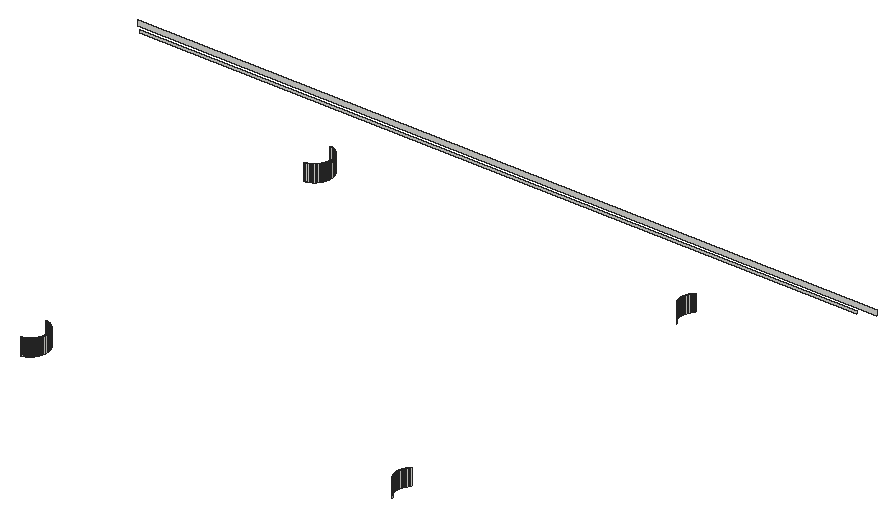
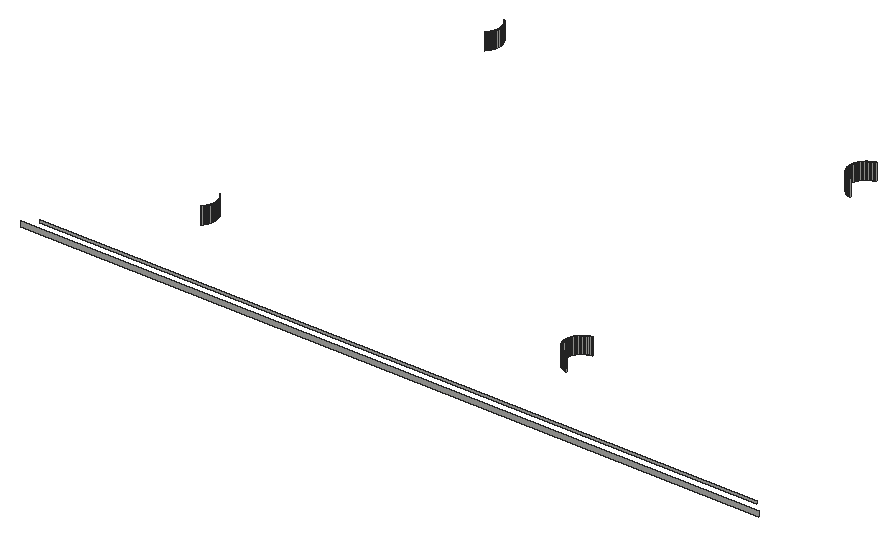
# SketchUp Ruby script. Lengths in inches.
U = 1.inch
M = Sketchup.active_model
def pt(a) = Geom::Point3d.new(a.map { |v| v * U })
def face(e, loops, mat)
  f = e.add_face(loops[0].map { |a| pt(a) })
  loops[1..].each { |l| e.add_face(l.map { |a| pt(a) }).erase! }
  f.material = f.back_material = mat if mat
  f
end
# faces: each face lists its corners as indices into pts; further lists are holes
def faces(e, pts, list, mat = nil) = list.each { |f| face(e, (f[0].is_a?(Array) ? f : [f]).map { |l| l.map { |i| pts[i] } }, mat) }
# xy, xz, yz: faces in a plane at the given z, y or x. An outline is a flat list of corners, or four numbers for a rectangle; further outlines are holes
def ring(l) = l.size == 4 ? [[l[0], l[1]], [l[2], l[1]], [l[2], l[3]], [l[0], l[3]]] : l.each_slice(2).to_a
def flat(e, list, mat, &to3) = list.each { |f| face(e, (f[0].is_a?(Array) ? f : [f]).map { |l| ring(l).map { |u, v| to3.(u, v) } }, mat) }
def xy(e, z, list, mat = nil) = flat(e, list, mat) { |x, y| [x, y, z] }
def xz(e, y, list, mat = nil) = flat(e, list, mat) { |x, z| [x, y, z] }
def yz(e, x, list, mat = nil) = flat(e, list, mat) { |y, z| [x, y, z] }
def lines(e, pts, list) = list.each { |a, b| e.add_line(pt(pts[a]), pt(pts[b])) }
# prism: a flat outline (further loops are holes) pulled along v
def prism(e, loops, v, mat = nil)
  f = face(e, loops, mat); d = Geom::Vector3d.new(v.map { |x| x * U })
  f.pushpull(f.normal.samedirection?(d) ? d.length : -d.length)
end
def box(e, o, s, mat = nil) = prism(e, [[o, [o[0] + s[0], o[1], o[2]], [o[0] + s[0], o[1] + s[1], o[2]], [o[0], o[1] + s[1], o[2]]]], [0, 0, s[2]], mat)
def at(x, y, z, deg = 0) = Geom::Transformation.translation(pt([x, y, z])) * Geom::Transformation.rotation(ORIGIN, Z_AXIS, deg.degrees)
def axes(o, x, y, z) = Geom::Transformation.new([*x, 0, *y, 0, *z, 0, *pt(o).to_a, 1])
def part(name) = M.definitions.add(name)
# library, detail: a bought-in or finely detailed component or shape, given as its bounding box
def library(name, o, s) = part(name).tap { |d| box(d.entities, o, s) }
def detail(e, o, s) = box(e.add_group.entities, o, s)
def put(e, d, t, mat = nil) = e.add_instance(d, t).tap { |i| i.material = mat if mat }
def group(e, t, mat = nil) = e.add_group.tap { |g| g.transformation = t; g.material = mat if mat }.entities
root = M.entities
xz(root,333,[[215,108,345,108.5]])
xz(root,335,[[213,107.5,347,108.5]])
yz(root,262.5,[[252.34,108,252.42,111],[252.42,108,252.5,111],[252.5,108,252.58,111],[252.58,108,252.66,111],[316.84,108,316.92,111],
  [316.92,108,317,111],[317,108,317.08,111],[317.08,108,317.16,111]])
yz(root,326,[[252.34,108,252.42,111],[252.42,108,252.5,111],[252.5,108,252.58,111],[252.58,108,252.66,111],[316.84,108,316.92,111],
  [316.92,108,317,111],[317,108,317.08,111],[317.08,108,317.16,111]])
p = [[260.125,249.57,108],[260.05,249.55,108],[260.05,249.55,111],[260.125,249.57,111],[260.2,249.58,108],[260.2,249.58,111],
  [260.28,249.6,108],[260.28,249.6,111],[260.35,249.625,108],[260.35,249.625,111],[260.43,249.65,108],[260.43,249.65,111],
  [260.5,249.67,108],[260.5,249.67,111],[260.58,249.7,108],[260.58,249.7,111],[260.65,249.73,108],[260.65,249.73,111],
  [260.72,249.76,108],[260.72,249.76,111],[260.79,249.79,108],[260.79,249.79,111],[260.86,249.83,108],[260.86,249.83,111],
  [260.93,249.86,108],[260.93,249.86,111],[261,249.9,108],[261,249.9,111],[261.07,249.94,108],[261.07,249.94,111],
  [261.13,249.98,108],[261.13,249.98,111],[261.2,250.03,108],[261.2,250.03,111],[261.26,250.07,108],[261.26,250.07,111],
  [261.33,250.12,108],[261.33,250.12,111],[261.39,250.17,108],[261.39,250.17,111],[261.45,250.22,108],[261.45,250.22,111],
  [261.51,250.27,108],[261.51,250.27,111],[261.57,250.32,108],[261.57,250.32,111],[261.62,250.38,108],[261.62,250.38,111],
  [326.93,250.32,108],[326.88,250.38,108],[326.88,250.38,111],[326.93,250.32,111],[261.68,250.43,108],[261.68,250.43,111],
  [261.73,250.49,108],[261.73,250.49,111],[326.82,250.43,108],[326.77,250.49,108],[326.77,250.49,111],[326.82,250.43,111],
  [261.78,250.55,108],[261.78,250.55,111],[326.72,250.55,108],[326.72,250.55,111],[261.83,250.61,108],[261.83,250.61,111],
  [261.88,250.67,108],[261.88,250.67,111],[326.67,250.61,108],[326.62,250.67,108],[326.62,250.67,111],[326.67,250.61,111],
  [261.93,250.74,108],[261.93,250.74,111],[261.97,250.8,108],[261.97,250.8,111],[326.57,250.74,108],[326.53,250.8,108],
  [326.53,250.8,111],[326.57,250.74,111],[262.02,250.87,108],[262.02,250.87,111],[326.48,250.87,108],[326.48,250.87,111],
  [262.06,250.93,108],[262.06,250.93,111],[262.1,251,108],[262.1,251,111],[326.44,250.93,108],[326.4,251,108],
  [326.4,251,111],[326.44,250.93,111],[262.14,251.07,108],[262.14,251.07,111],[326.36,251.07,108],[326.36,251.07,111],
  [262.17,251.14,108],[262.17,251.14,111],[262.21,251.21,108],[262.21,251.21,111],[326.33,251.14,108],[326.29,251.21,108],
  [326.29,251.21,111],[326.33,251.14,111],[262.24,251.28,108],[262.24,251.28,111],[326.26,251.28,108],[326.26,251.28,111],
  [262.27,251.35,108],[262.27,251.35,111],[326.23,251.35,108],[326.23,251.35,111],[262.3,251.42,108],[262.3,251.42,111],
  [262.33,251.5,108],[262.33,251.5,111],[326.2,251.42,108],[326.17,251.5,108],[326.17,251.5,111],[326.2,251.42,111],
  [262.35,251.57,108],[262.35,251.57,111],[326.15,251.57,108],[326.15,251.57,111],[262.375,251.65,108],[262.375,251.65,111],
  [262.4,251.72,108],[262.4,251.72,111],[326.125,251.65,108],[326.1,251.72,108],[326.1,251.72,111],[326.125,251.65,111],
  [262.42,251.8,108],[262.42,251.8,111],[326.08,251.8,108],[326.08,251.8,111],[262.43,251.875,108],[262.43,251.875,111],
  [326.07,251.875,108],[326.07,251.875,111],[262.45,251.95,108],[262.45,251.95,111],[326.05,251.95,108],[326.05,251.95,111],
  [262.46,252.03,108],[262.46,252.03,111],[262.47,252.11,108],[262.47,252.11,111],[326.04,252.03,108],[326.03,252.11,108],
  [326.03,252.11,111],[326.04,252.03,111],[262.48,252.1875,108],[262.48,252.1875,111],[326.02,252.1875,108],[326.02,252.1875,111],
  [262.49,252.26,108],[262.49,252.26,111],[326.01,252.26,108],[326.01,252.26,111],[262.5,252.34,108],[262.5,252.34,111],
  [326,252.34,108],[326,252.34,111],[262.48,252.8125,108],[262.49,252.74,108],[262.49,252.74,111],[262.48,252.8125,111],
  [262.5,252.66,108],[262.5,252.66,111],[326,252.66,108],[326.01,252.74,108],[326.01,252.74,111],[326,252.66,111],
  [326.02,252.8125,108],[326.02,252.8125,111],[262.47,252.89,108],[262.47,252.89,111],[326.03,252.89,108],[326.03,252.89,111],
  [262.46,252.97,108],[262.46,252.97,111],[326.04,252.97,108],[326.04,252.97,111],[262.43,253.125,108],[262.45,253.05,108],
  [262.45,253.05,111],[262.43,253.125,111],[326.05,253.05,108],[326.05,253.05,111],[326.07,253.125,108],[326.07,253.125,111],
  [262.42,253.2,108],[262.42,253.2,111],[326.08,253.2,108],[326.08,253.2,111],[262.4,253.28,108],[262.4,253.28,111],
  [326.1,253.28,108],[326.1,253.28,111],[262.375,253.35,108],[262.375,253.35,111],[326.125,253.35,108],[326.125,253.35,111],
  [262.33,253.5,108],[262.35,253.43,108],[262.35,253.43,111],[262.33,253.5,111],[326.15,253.43,108],[326.15,253.43,111],
  [326.17,253.5,108],[326.17,253.5,111],[262.3,253.58,108],[262.3,253.58,111],[326.2,253.58,108],[326.2,253.58,111],
  [262.24,253.72,108],[262.27,253.65,108],[262.27,253.65,111],[262.24,253.72,111],[326.23,253.65,108],[326.23,253.65,111],
  [326.26,253.72,108],[326.26,253.72,111],[262.21,253.79,108],[262.21,253.79,111],[326.29,253.79,108],[326.29,253.79,111],
  [262.17,253.86,108],[262.17,253.86,111],[326.33,253.86,108],[326.33,253.86,111],[262.1,254,108],[262.14,253.93,108],
  [262.14,253.93,111],[262.1,254,111],[326.36,253.93,108],[326.36,253.93,111],[326.4,254,108],[326.4,254,111],
  [262.06,254.07,108],[262.06,254.07,111],[326.44,254.07,108],[326.44,254.07,111],[261.97,254.2,108],[262.02,254.13,108],
  [262.02,254.13,111],[261.97,254.2,111],[326.48,254.13,108],[326.48,254.13,111],[326.53,254.2,108],[326.53,254.2,111],
  [261.93,254.26,108],[261.93,254.26,111],[326.57,254.26,108],[326.57,254.26,111],[261.83,254.39,108],[261.88,254.33,108],
  [261.88,254.33,111],[261.83,254.39,111],[326.62,254.33,108],[326.62,254.33,111],[326.67,254.39,108],[326.67,254.39,111],
  [261.73,254.51,108],[261.78,254.45,108],[261.78,254.45,111],[261.73,254.51,111],[326.72,254.45,108],[326.72,254.45,111],
  [326.77,254.51,108],[326.77,254.51,111],[261.68,254.57,108],[261.68,254.57,111],[326.82,254.57,108],[326.82,254.57,111],
  [261.57,254.68,108],[261.62,254.62,108],[261.62,254.62,111],[261.57,254.68,111],[326.88,254.62,108],[326.88,254.62,111],
  [326.93,254.68,108],[326.93,254.68,111],[261.45,254.78,108],[261.51,254.73,108],[261.51,254.73,111],[261.45,254.78,111],
  [261.33,254.88,108],[261.39,254.83,108],[261.39,254.83,111],[261.33,254.88,111],[261.2,254.97,108],[261.26,254.93,108],
  [261.26,254.93,111],[261.2,254.97,111],[261.07,255.06,108],[261.13,255.02,108],[261.13,255.02,111],[261.07,255.06,111],
  [260.86,255.17,108],[260.93,255.14,108],[260.93,255.14,111],[260.86,255.17,111],[261,255.1,108],[261,255.1,111],
  [260.65,255.27,108],[260.72,255.24,108],[260.72,255.24,111],[260.65,255.27,111],[260.79,255.21,108],[260.79,255.21,111],
  [260.43,255.35,108],[260.5,255.33,108],[260.5,255.33,111],[260.43,255.35,111],[260.58,255.3,108],[260.58,255.3,111],
  [259.97,255.46,108],[260.05,255.45,108],[260.05,255.45,111],[259.97,255.46,111],[260.125,255.43,108],[260.125,255.43,111],
  [260.2,255.42,108],[260.2,255.42,111],[260.28,255.4,108],[260.28,255.4,111],[260.35,255.375,108],[260.35,255.375,111],
  [259.97,314.04,108],[259.89,314.03,108],[259.89,314.03,111],[259.97,314.04,111],[260.05,314.05,108],[260.05,314.05,111],
  [260.125,314.07,108],[260.125,314.07,111],[260.2,314.08,108],[260.2,314.08,111],[260.28,314.1,108],[260.28,314.1,111],
  [260.35,314.125,108],[260.35,314.125,111],[260.43,314.15,108],[260.43,314.15,111],[260.5,314.17,108],[260.5,314.17,111],
  [260.58,314.2,108],[260.58,314.2,111],[260.65,314.23,108],[260.65,314.23,111],[260.72,314.26,108],[260.72,314.26,111],
  [260.79,314.29,108],[260.79,314.29,111],[260.86,314.33,108],[260.86,314.33,111],[260.93,314.36,108],[260.93,314.36,111],
  [261,314.4,108],[261,314.4,111],[261.07,314.44,108],[261.07,314.44,111],[261.13,314.48,108],[261.13,314.48,111],
  [261.2,314.53,108],[261.2,314.53,111],[261.26,314.57,108],[261.26,314.57,111],[261.33,314.62,108],[261.33,314.62,111],
  [261.39,314.67,108],[261.39,314.67,111],[261.45,314.72,108],[261.45,314.72,111],[261.51,314.77,108],[261.51,314.77,111],
  [261.57,314.82,108],[261.57,314.82,111],[261.62,314.88,108],[261.62,314.88,111],[326.93,314.82,108],[326.88,314.88,108],
  [326.88,314.88,111],[326.93,314.82,111],[261.68,314.93,108],[261.68,314.93,111],[261.73,314.99,108],[261.73,314.99,111],
  [326.82,314.93,108],[326.77,314.99,108],[326.77,314.99,111],[326.82,314.93,111],[261.78,315.05,108],[261.78,315.05,111],
  [326.72,315.05,108],[326.72,315.05,111],[261.83,315.11,108],[261.83,315.11,111],[261.88,315.17,108],[261.88,315.17,111],
  [326.67,315.11,108],[326.62,315.17,108],[326.62,315.17,111],[326.67,315.11,111],[261.93,315.24,108],[261.93,315.24,111],
  [261.97,315.3,108],[261.97,315.3,111],[326.57,315.24,108],[326.53,315.3,108],[326.53,315.3,111],[326.57,315.24,111],
  [262.02,315.37,108],[262.02,315.37,111],[326.48,315.37,108],[326.48,315.37,111],[262.06,315.43,108],[262.06,315.43,111],
  [262.1,315.5,108],[262.1,315.5,111],[326.44,315.43,108],[326.4,315.5,108],[326.4,315.5,111],[326.44,315.43,111],
  [262.14,315.57,108],[262.14,315.57,111],[326.36,315.57,108],[326.36,315.57,111],[262.17,315.64,108],[262.17,315.64,111],
  [262.21,315.71,108],[262.21,315.71,111],[326.33,315.64,108],[326.29,315.71,108],[326.29,315.71,111],[326.33,315.64,111],
  [262.24,315.78,108],[262.24,315.78,111],[326.26,315.78,108],[326.26,315.78,111],[262.27,315.85,108],[262.27,315.85,111],
  [326.23,315.85,108],[326.23,315.85,111],[262.3,315.92,108],[262.3,315.92,111],[262.33,316,108],[262.33,316,111],
  [326.2,315.92,108],[326.17,316,108],[326.17,316,111],[326.2,315.92,111],[262.35,316.07,108],[262.35,316.07,111],
  [326.15,316.07,108],[326.15,316.07,111],[262.375,316.15,108],[262.375,316.15,111],[262.4,316.22,108],[262.4,316.22,111],
  [326.125,316.15,108],[326.1,316.22,108],[326.1,316.22,111],[326.125,316.15,111],[262.42,316.3,108],[262.42,316.3,111],
  [326.08,316.3,108],[326.08,316.3,111],[262.43,316.375,108],[262.43,316.375,111],[326.07,316.375,108],[326.07,316.375,111],
  [262.45,316.45,108],[262.45,316.45,111],[326.05,316.45,108],[326.05,316.45,111],[262.46,316.53,108],[262.46,316.53,111],
  [262.47,316.61,108],[262.47,316.61,111],[326.04,316.53,108],[326.03,316.61,108],[326.03,316.61,111],[326.04,316.53,111],
  [262.48,316.6875,108],[262.48,316.6875,111],[326.02,316.6875,108],[326.02,316.6875,111],[262.49,316.76,108],[262.49,316.76,111],
  [326.01,316.76,108],[326.01,316.76,111],[262.5,316.84,108],[262.5,316.84,111],[326,316.84,108],[326,316.84,111],
  [262.48,317.3125,108],[262.49,317.24,108],[262.49,317.24,111],[262.48,317.3125,111],[262.5,317.16,108],[262.5,317.16,111],
  [326,317.16,108],[326.01,317.24,108],[326.01,317.24,111],[326,317.16,111],[326.02,317.3125,108],[326.02,317.3125,111],
  [262.47,317.39,108],[262.47,317.39,111],[326.03,317.39,108],[326.03,317.39,111],[262.46,317.47,108],[262.46,317.47,111],
  [326.04,317.47,108],[326.04,317.47,111],[262.43,317.625,108],[262.45,317.55,108],[262.45,317.55,111],[262.43,317.625,111],
  [326.05,317.55,108],[326.05,317.55,111],[326.07,317.625,108],[326.07,317.625,111],[262.42,317.7,108],[262.42,317.7,111],
  [326.08,317.7,108],[326.08,317.7,111],[262.4,317.78,108],[262.4,317.78,111],[326.1,317.78,108],[326.1,317.78,111],
  [262.375,317.85,108],[262.375,317.85,111],[326.125,317.85,108],[326.125,317.85,111],[262.33,318,108],[262.35,317.93,108],
  [262.35,317.93,111],[262.33,318,111],[326.15,317.93,108],[326.15,317.93,111],[326.17,318,108],[326.17,318,111],
  [262.3,318.08,108],[262.3,318.08,111],[326.2,318.08,108],[326.2,318.08,111],[262.24,318.22,108],[262.27,318.15,108],
  [262.27,318.15,111],[262.24,318.22,111],[326.23,318.15,108],[326.23,318.15,111],[326.26,318.22,108],[326.26,318.22,111],
  [262.21,318.29,108],[262.21,318.29,111],[326.29,318.29,108],[326.29,318.29,111],[262.17,318.36,108],[262.17,318.36,111],
  [326.33,318.36,108],[326.33,318.36,111],[262.1,318.5,108],[262.14,318.43,108],[262.14,318.43,111],[262.1,318.5,111],
  [326.36,318.43,108],[326.36,318.43,111],[326.4,318.5,108],[326.4,318.5,111],[262.06,318.57,108],[262.06,318.57,111],
  [326.44,318.57,108],[326.44,318.57,111],[261.97,318.7,108],[262.02,318.63,108],[262.02,318.63,111],[261.97,318.7,111],
  [326.48,318.63,108],[326.48,318.63,111],[326.53,318.7,108],[326.53,318.7,111],[261.93,318.76,108],[261.93,318.76,111],
  [326.57,318.76,108],[326.57,318.76,111],[261.83,318.89,108],[261.88,318.83,108],[261.88,318.83,111],[261.83,318.89,111],
  [326.62,318.83,108],[326.62,318.83,111],[326.67,318.89,108],[326.67,318.89,111],[261.73,319.01,108],[261.78,318.95,108],
  [261.78,318.95,111],[261.73,319.01,111],[326.72,318.95,108],[326.72,318.95,111],[326.77,319.01,108],[326.77,319.01,111],
  [261.68,319.07,108],[261.68,319.07,111],[326.82,319.07,108],[326.82,319.07,111],[261.57,319.18,108],[261.62,319.12,108],
  [261.62,319.12,111],[261.57,319.18,111],[326.88,319.12,108],[326.88,319.12,111],[326.93,319.18,108],[326.93,319.18,111],
  [261.45,319.28,108],[261.51,319.23,108],[261.51,319.23,111],[261.45,319.28,111],[261.33,319.38,108],[261.39,319.33,108],
  [261.39,319.33,111],[261.33,319.38,111],[261.2,319.47,108],[261.26,319.43,108],[261.26,319.43,111],[261.2,319.47,111],
  [261.07,319.56,108],[261.13,319.52,108],[261.13,319.52,111],[261.07,319.56,111],[260.86,319.67,108],[260.93,319.64,108],
  [260.93,319.64,111],[260.86,319.67,111],[261,319.6,108],[261,319.6,111],[260.65,319.77,108],[260.72,319.74,108],
  [260.72,319.74,111],[260.65,319.77,111],[260.79,319.71,108],[260.79,319.71,111],[260.43,319.85,108],[260.5,319.83,108],
  [260.5,319.83,111],[260.43,319.85,111],[260.58,319.8,108],[260.58,319.8,111],[259.97,319.96,108],[260.05,319.95,108],
  [260.05,319.95,111],[259.97,319.96,111],[260.125,319.93,108],[260.125,319.93,111],[260.2,319.92,108],[260.2,319.92,111],
  [260.28,319.9,108],[260.28,319.9,111],[260.35,319.875,108],[260.35,319.875,111],[259.89,319.97,108],[259.89,319.97,111]]
faces(root,p,[[0,1,2,3],[4,0,3,5],[6,4,5,7],[8,6,7,9],[10,8,9,11],[12,10,11,13],[14,12,13,15],[16,14,15,17],
  [18,16,17,19],[20,18,19,21],[22,20,21,23],[24,22,23,25],[26,24,25,27],[28,26,27,29],[30,28,29,31],[32,30,31,33],
  [34,32,33,35],[36,34,35,37],[38,36,37,39],[40,38,39,41],[42,40,41,43],[44,42,43,45],[46,44,45,47],[48,49,50,51],
  [52,46,47,53],[54,52,53,55],[56,57,58,59],[49,56,59,50],[60,54,55,61],[57,62,63,58],[64,60,61,65],[66,64,65,67],
  [68,69,70,71],[62,68,71,63],[72,66,67,73],[74,72,73,75],[76,77,78,79],[69,76,79,70],[80,74,75,81],[77,82,83,78],
  [84,80,81,85],[86,84,85,87],[88,89,90,91],[82,88,91,83],[92,86,87,93],[89,94,95,90],[96,92,93,97],[98,96,97,99],
  [100,101,102,103],[94,100,103,95],[104,98,99,105],[101,106,107,102],[108,104,105,109],[106,110,111,107],[112,108,109,113],[114,112,113,115],
  [116,117,118,119],[110,116,119,111],[120,114,115,121],[117,122,123,118],[124,120,121,125],[126,124,125,127],[128,129,130,131],[122,128,131,123],
  [132,126,127,133],[129,134,135,130],[136,132,133,137],[134,138,139,135],[140,136,137,141],[138,142,143,139],[144,140,141,145],[146,144,145,147],
  [148,149,150,151],[142,148,151,143],[152,146,147,153],[149,154,155,150],[156,152,153,157],[154,158,159,155],[160,156,157,161],[158,162,163,159],
  [164,165,166,167],[165,168,169,166],[170,171,172,173],[171,174,175,172],[176,164,167,177],[174,178,179,175],[180,176,177,181],[178,182,183,179],
  [184,185,186,187],[185,180,181,186],[182,188,189,183],[188,190,191,189],[192,184,187,193],[190,194,195,191],[196,192,193,197],[194,198,199,195],
  [200,196,197,201],[198,202,203,199],[204,205,206,207],[205,200,201,206],[202,208,209,203],[208,210,211,209],[212,204,207,213],[210,214,215,211],
  [216,217,218,219],[217,212,213,218],[214,220,221,215],[220,222,223,221],[224,216,219,225],[222,226,227,223],[228,224,225,229],[226,230,231,227],
  [232,233,234,235],[233,228,229,234],[230,236,237,231],[236,238,239,237],[240,232,235,241],[238,242,243,239],[244,245,246,247],[245,240,241,246],
  [242,248,249,243],[248,250,251,249],[252,244,247,253],[250,254,255,251],[256,257,258,259],[257,252,253,258],[254,260,261,255],[260,262,263,261],
  [264,265,266,267],[265,256,259,266],[262,268,269,263],[268,270,271,269],[272,264,267,273],[270,274,275,271],[276,277,278,279],[277,272,273,278],
  [274,280,281,275],[280,282,283,281],[284,285,286,287],[285,276,279,286],[288,289,290,291],[289,284,287,290],[292,293,294,295],[293,288,291,294],
  [296,297,298,299],[297,292,295,298],[300,301,302,303],[301,304,305,302],[304,296,299,305],[306,307,308,309],[307,310,311,308],[310,300,303,311],
  [312,313,314,315],[313,316,317,314],[316,306,309,317],[318,319,320,321],[319,322,323,320],[322,324,325,323],[324,326,327,325],[326,328,329,327],
  [328,312,315,329],[330,331,332,333],[334,330,333,335],[336,334,335,337],[338,336,337,339],[340,338,339,341],[342,340,341,343],[344,342,343,345],
  [346,344,345,347],[348,346,347,349],[350,348,349,351],[352,350,351,353],[354,352,353,355],[356,354,355,357],[358,356,357,359],[360,358,359,361],
  [362,360,361,363],[364,362,363,365],[366,364,365,367],[368,366,367,369],[370,368,369,371],[372,370,371,373],[374,372,373,375],[376,374,375,377],
  [378,376,377,379],[380,378,379,381],[382,383,384,385],[386,380,381,387],[388,386,387,389],[390,391,392,393],[383,390,393,384],[394,388,389,395],
  [391,396,397,392],[398,394,395,399],[400,398,399,401],[402,403,404,405],[396,402,405,397],[406,400,401,407],[408,406,407,409],[410,411,412,413],
  [403,410,413,404],[414,408,409,415],[411,416,417,412],[418,414,415,419],[420,418,419,421],[422,423,424,425],[416,422,425,417],[426,420,421,427],
  [423,428,429,424],[430,426,427,431],[432,430,431,433],[434,435,436,437],[428,434,437,429],[438,432,433,439],[435,440,441,436],[442,438,439,443],
  [440,444,445,441],[446,442,443,447],[448,446,447,449],[450,451,452,453],[444,450,453,445],[454,448,449,455],[451,456,457,452],[458,454,455,459],
  [460,458,459,461],[462,463,464,465],[456,462,465,457],[466,460,461,467],[463,468,469,464],[470,466,467,471],[468,472,473,469],[474,470,471,475],
  [472,476,477,473],[478,474,475,479],[480,478,479,481],[482,483,484,485],[476,482,485,477],[486,480,481,487],[483,488,489,484],[490,486,487,491],
  [488,492,493,489],[494,490,491,495],[492,496,497,493],[498,499,500,501],[499,502,503,500],[504,505,506,507],[505,508,509,506],[510,498,501,511],
  [508,512,513,509],[514,510,511,515],[512,516,517,513],[518,519,520,521],[519,514,515,520],[516,522,523,517],[522,524,525,523],[526,518,521,527],
  [524,528,529,525],[530,526,527,531],[528,532,533,529],[534,530,531,535],[532,536,537,533],[538,539,540,541],[539,534,535,540],[536,542,543,537],
  [542,544,545,543],[546,538,541,547],[544,548,549,545],[550,551,552,553],[551,546,547,552],[548,554,555,549],[554,556,557,555],[558,550,553,559],
  [556,560,561,557],[562,558,559,563],[560,564,565,561],[566,567,568,569],[567,562,563,568],[564,570,571,565],[570,572,573,571],[574,566,569,575],
  [572,576,577,573],[578,579,580,581],[579,574,575,580],[576,582,583,577],[582,584,585,583],[586,578,581,587],[584,588,589,585],[590,591,592,593],
  [591,586,587,592],[588,594,595,589],[594,596,597,595],[598,599,600,601],[599,590,593,600],[596,602,603,597],[602,604,605,603],[606,598,601,607],
  [604,608,609,605],[610,611,612,613],[611,606,607,612],[608,614,615,609],[614,616,617,615],[618,619,620,621],[619,610,613,620],[622,623,624,625],
  [623,618,621,624],[626,627,628,629],[627,622,625,628],[630,631,632,633],[631,626,629,632],[634,635,636,637],[635,638,639,636],[638,630,633,639],
  [640,641,642,643],[641,644,645,642],[644,634,637,645],[646,647,648,649],[647,650,651,648],[650,640,643,651],[652,653,654,655],[653,656,657,654],
  [656,658,659,657],[658,660,661,659],[660,662,663,661],[662,646,649,663],[664,652,655,665]])
